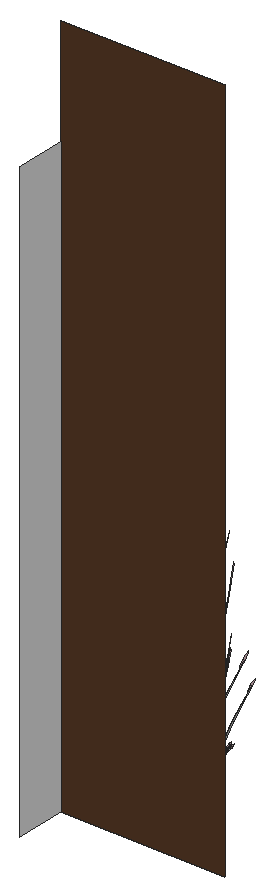
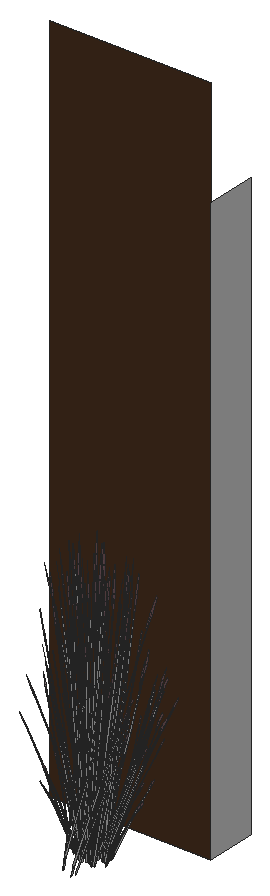
# SketchUp Ruby script. Lengths in inches.
U = 1.inch
M = Sketchup.active_model
def pt(a) = Geom::Point3d.new(a.map { |v| v * U })
def face(e, loops, mat)
  f = e.add_face(loops[0].map { |a| pt(a) })
  loops[1..].each { |l| e.add_face(l.map { |a| pt(a) }).erase! }
  f.material = f.back_material = mat if mat
  f
end
# faces: each face lists its corners as indices into pts; further lists are holes
def faces(e, pts, list, mat = nil) = list.each { |f| face(e, (f[0].is_a?(Array) ? f : [f]).map { |l| l.map { |i| pts[i] } }, mat) }
# xy, xz, yz: faces in a plane at the given z, y or x. An outline is a flat list of corners, or four numbers for a rectangle; further outlines are holes
def ring(l) = l.size == 4 ? [[l[0], l[1]], [l[2], l[1]], [l[2], l[3]], [l[0], l[3]]] : l.each_slice(2).to_a
def flat(e, list, mat, &to3) = list.each { |f| face(e, (f[0].is_a?(Array) ? f : [f]).map { |l| ring(l).map { |u, v| to3.(u, v) } }, mat) }
def xy(e, z, list, mat = nil) = flat(e, list, mat) { |x, y| [x, y, z] }
def xz(e, y, list, mat = nil) = flat(e, list, mat) { |x, z| [x, y, z] }
def yz(e, x, list, mat = nil) = flat(e, list, mat) { |y, z| [x, y, z] }
def lines(e, pts, list) = list.each { |a, b| e.add_line(pt(pts[a]), pt(pts[b])) }
# prism: a flat outline (further loops are holes) pulled along v
def prism(e, loops, v, mat = nil)
  f = face(e, loops, mat); d = Geom::Vector3d.new(v.map { |x| x * U })
  f.pushpull(f.normal.samedirection?(d) ? d.length : -d.length)
end
def box(e, o, s, mat = nil) = prism(e, [[o, [o[0] + s[0], o[1], o[2]], [o[0] + s[0], o[1] + s[1], o[2]], [o[0], o[1] + s[1], o[2]]]], [0, 0, s[2]], mat)
def at(x, y, z, deg = 0) = Geom::Transformation.translation(pt([x, y, z])) * Geom::Transformation.rotation(ORIGIN, Z_AXIS, deg.degrees)
def axes(o, x, y, z) = Geom::Transformation.new([*x, 0, *y, 0, *z, 0, *pt(o).to_a, 1])
def part(name) = M.definitions.add(name)
# library, detail: a bought-in or finely detailed component or shape, given as its bounding box
def library(name, o, s) = part(name).tap { |d| box(d.entities, o, s) }
def detail(e, o, s) = box(e.add_group.entities, o, s)
def put(e, d, t, mat = nil) = e.add_instance(d, t).tap { |i| i.material = mat if mat }
def group(e, t, mat = nil) = e.add_group.tap { |g| g.transformation = t; g.material = mat if mat }.entities
root = M.entities
M.materials.add("LightPink_Translucent").color = [144, 107, 117]
M.materials["LightPink_Translucent"].alpha = 0.75
M.materials.add("Wood_Veneer_15_1K").color = [81, 54, 35]
M.materials.add("[_0053_Ivory_]").color = [200, 200, 200]
c1 = part("blade")
p = [[2.15,0.21,22],[0,0.17,0],[0.09,0.45,0],[2.18,0.31,22],[2.29,0.31,22],[0.38,0.45,0],
  [2.48,0.24,33],[2.49,0.24,33],[2.48,0.22,33]]
faces(c1.entities,p,[[0,1,2,3],[4,5,2,3],[6,3,4,7],[8,0,3,6]])
c2 = part("seeds")
p = [[0.3,-0.1,1.38],[-0.01,-0.03,1.59],[-0.01,-0.03,0.03],[0.14,-0.07,-0.07],[0.29,-0.03,3],[0.15,0.01,3.11]]
faces(c2.entities,p,[[0,1,2,3],[1,0,4,5]],"LightPink_Translucent")
c3 = part("blade with seeds")
put(c3.entities,c1,at(0,0,0))
put(c3.entities,c2,axes([2.4,0.25,30.99],[1.5799,-0.05474,1.17369],[-0.12525,1.92788,0.29478],[-0.07173,-0.02425,1.56792]))
xz(root,269.15,[[617.51,252,653.51,408]],"Wood_Veneer_15_1K")
yz(root,617.51,[[257.92,252,269.15,384]],"[_0053_Ivory_]")
put(root,c3,axes([630.49,281.87,255.53],[0.13883,0.2019,1.71376],[-0.64153,0.16998,0.13857],[-0.14499,-0.31697,0.73262]),"[_0053_Ivory_]")
put(root,c3,axes([632.98,281.57,254.24],[-0.17264,0.12729,1.43002],[-0.51703,-0.22279,-0.30754],[0.09584,-0.27707,0.61141]),"[_0053_Ivory_]")
put(root,c3,axes([632.2,282.02,256.63],[-0.28988,-0.51132,-0.71045],[0.59671,-0.28496,0.08574],[-0.06778,-0.24706,1.00501]),"[_0053_Ivory_]")
put(root,c3,axes([630.3125,281.33,254.24],[-0.03678,0.20572,1.43002],[-0.53767,0.17221,-0.30754],[-0.12568,-0.26589,0.61141]),"[_0053_Ivory_]")
put(root,c3,axes([631.7,280.88,253.15],[-0.10187,0.02266,1.76342],[-0.56336,-0.25503,-0.26939],[0.00945,-0.21273,0.30037]),"[_0053_Ivory_]")
put(root,c3,axes([633.4,282.52,256.63],[0.0158,-0.58168,-0.71045],[0.66548,0.03907,0.08574],[0.07023,-0.24643,1.00501]),"[_0053_Ivory_]")
put(root,c3,axes([632.25,281.58,256.18],[0.1831,-0.48359,-0.35414],[0.53419,0.14105,0.4572],[-0.04898,-0.1947,0.87481]),"[_0053_Ivory_]")
put(root,c3,axes([632.65,282.22,255.53],[-0.11309,0.21615,1.71376],[-0.47441,-0.44731,0.13857],[0.21402,-0.27879,0.73262]),"[_0053_Ivory_]")
put(root,c3,axes([631.98,281.91,256.33],[-0.59704,-0.15764,-0.51099],[0.20464,-0.54049,-0.3958],[-0.05475,-0.21761,0.97773]),"[_0053_Ivory_]")
put(root,c3,axes([632.35,280.5625,254.42],[0.07791,0.3667,1.1486],[-0.43222,-0.2031,0.84392],[0.04651,-0.18776,0.25299]),"[_0053_Ivory_]")
put(root,c3,axes([633.27,282.32,256.33],[-0.43478,-0.42253,-0.51099],[0.45929,-0.37004,-0.3958],[0.06615,-0.21468,0.97773]),"[_0053_Ivory_]")
put(root,c3,axes([633.68,282.17,256.18],[0.41095,-0.33109,-0.35414],[0.38901,0.37805,0.4572],[0.05919,-0.19208,0.87481]),"[_0053_Ivory_]")
put(root,c3,axes([630.125,281,254.42],[0.31682,0.21887,1.1486],[-0.4614,0.13157,0.84392],[-0.09872,-0.16821,0.25299]),"[_0053_Ivory_]")
put(root,c3,axes([630.89,282.16,256.63],[-0.51789,-0.30395,-0.71045],[0.36805,-0.53263,0.08574],[-0.18764,-0.18149,1.00501]),"[_0053_Ivory_]")
put(root,c3,axes([630.71,281.76,256.18],[-0.0938,-0.50652,-0.35414],[0.53623,-0.13375,0.4572],[-0.14403,-0.14515,0.87481]),"[_0053_Ivory_]")
put(root,c3,axes([629.875,281.66,253.15],[-0.05883,0.08284,1.76342],[-0.59454,0.17861,-0.26939],[-0.14363,-0.16248,0.30037]),"[_0053_Ivory_]")
put(root,c3,axes([630.86,283.9375,253.75],[-0.24943,-0.64486,-0.69835],[0.71849,-0.23224,-0.18329],[-0.02757,-0.21836,1.54149]),"[_0053_Ivory_]")
put(root,c3,axes([629.56,282.5,255.53],[0.2256,0.10835,1.71376],[-0.46687,0.45453,0.13857],[-0.29098,-0.20505,0.73262]),"[_0053_Ivory_]")
put(root,c3,axes([634.19,281.97,253.15],[-0.0909,-0.04954,1.76342],[-0.2335,-0.55347,-0.26939],[0.15752,-0.1502,0.30037]),"[_0053_Ivory_]")
put(root,c3,axes([630.65,282.18,256.33],[-0.59932,0.14948,-0.51099],[-0.10484,-0.56611,-0.3958],[-0.16097,-0.16223,0.97773]),"[_0053_Ivory_]")
put(root,c3,axes([634.1875,283.53,256.63],[0.31725,-0.49618,-0.71045],[0.55593,0.35263,0.08574],[0.18942,-0.17977,1.00501]),"[_0053_Ivory_]")
put(root,c3,axes([630.76,282.08,254.03],[-0.37973,-0.63014,0],[0.6353,-0.35142,-0.51607],[0.14469,-0.08004,1.63711]),"[_0053_Ivory_]")
put(root,c3,axes([634.17,283.3,256.33],[-0.15602,-0.5742,-0.51099],[0.59087,-0.10045,-0.3958],[0.16933,-0.15423,0.97773]),"[_0053_Ivory_]")
put(root,c3,axes([631.59,281.32,253.78],[-0.4197,0.36076,-0.03893],[-0.38456,-0.39511,-0.17649],[-0.02707,-0.11196,0.58215]),"[_0053_Ivory_]")
put(root,c3,axes([632.13,285.6,254.98],[0.52485,0.25358,1.51261],[-0.51417,0.54629,0.59816],[-0.23031,-0.32378,1.26806]),"[_0053_Ivory_]")
put(root,c3,axes([629.39,283.85,253.67],[0,-0.62885,-0.49651],[0.67951,0,0],[0,-0.14322,1.57504]),"[_0053_Ivory_]")
put(root,c3,axes([631.27,281.99,253.67],[0.56842,-0.31443,-0.49651],[0.33976,0.56381,0],[0.12946,-0.07161,1.57504]),"[_0053_Ivory_]")
put(root,c3,axes([634.65,283.07,254.24],[-0.21697,-0.01863,1.43002],[-0.22228,-0.49966,-0.30754],[0.26655,-0.14135,0.61141]),"[_0053_Ivory_]")
put(root,c3,axes([631.95,283.28,253.71],[0.40909,-0.47266,-0.62353],[0.50819,0.4286,-0.16365],[0.16393,-0.11791,1.37633]),"[_0053_Ivory_]")
put(root,c3,axes([634.9,282.15,254.42],[-0.2023,0.32011,1.1486],[-0.17388,-0.43009,0.84392],[0.16708,-0.10777,0.25299]),"[_0053_Ivory_]")
put(root,c3,axes([634.61,283.36,256.18],[0.52868,-0.08987,-0.35414],[0.1396,0.51376,0.4572],[0.1515,-0.13799,0.87481]),"[_0053_Ivory_]")
put(root,c3,axes([631.24,284.1,253.86],[0.29468,-0.56664,-0.44739],[0.61229,0.27271,0.21531],[0,-0.13062,1.43643]),"[_0053_Ivory_]")
put(root,c3,axes([629.47,282.65,256.18],[-0.34557,-0.39372,-0.35414],[0.39459,-0.37271,0.4572],[-0.20048,-0.05671,0.87481]),"[_0053_Ivory_]")
put(root,c3,axes([631.5,283.82,254.32],[-0.07077,-0.71755,-0.29095],[0.73712,-0.04339,-0.50002],[0.1298,-0.09558,1.59708]),"[_0053_Ivory_]")
put(root,c3,axes([629.68,283.86,253.68],[0.42396,-0.39235,-0.30978],[0.42396,0.39235,0.30978],[0,-0.12637,1.38974]),"[_0053_Ivory_]")
put(root,c3,axes([629.51,281.98,253.78],[-0.1752,0.51349,-0.03893],[-0.53924,-0.15795,-0.17649],[-0.08187,-0.08399,0.58215]),"[_0053_Ivory_]")
put(root,c3,axes([631.16,284.58,254.32],[-0.68399,-0.30005,-0.29095],[0.32934,-0.63331,-0.50002],[-0.0215,-0.15549,1.59708]),"[_0053_Ivory_]")
put(root,c3,axes([629.22,284.32,254.03],[-0.75945,0,0],[0,-0.70283,-0.51607],[0,-0.16007,1.63711]),"[_0053_Ivory_]")
put(root,c3,axes([629.35,283.07,254.24],[0.11858,0.17508,1.43002],[-0.27325,0.4759,-0.30754],[-0.28057,-0.11375,0.61141]),"[_0053_Ivory_]")
put(root,c3,axes([631.41,282.23,253.68],[0.56663,0.1556,-0.30978],[-0.14267,0.54795,0.30978],[0.11423,-0.06319,1.38974]),"[_0053_Ivory_]")
put(root,c3,axes([629.83,282.91,256.63],[-0.60713,-0.01514,-0.71045],[0.04078,-0.63759,0.08574],[-0.25721,-0.06729,1.00501]),"[_0053_Ivory_]")
put(root,c3,axes([629.8,284.14,253.98],[-0.56493,0.5287,0.30756],[-0.56528,-0.52313,-0.36492],[-0.01973,-0.15014,1.64885]),"[_0053_Ivory_]")
put(root,c3,axes([631.6,284.39,254.09],[0.68433,0.30479,0.24065],[-0.32934,0.63331,0.50002],[0,-0.14599,1.60543]),"[_0053_Ivory_]")
put(root,c3,axes([631.33,285.24,254.09],[0.16098,-0.74515,-0.23429],[0.76326,0.12989,0.51271],[-0.13337,-0.1029,1.5644]),"[_0053_Ivory_]")
put(root,c3,axes([629.63,283.04,256.33],[-0.44101,0.41656,-0.51099],[-0.38623,-0.44004,-0.3958],[-0.22407,-0.06338,0.97773]),"[_0053_Ivory_]")
put(root,c3,axes([628.64,283.59,254.42],[0.38775,-0.045,1.1486],[-0.24596,0.39648,0.84392],[-0.19161,-0.05948,0.25299]),"[_0053_Ivory_]")
put(root,c3,axes([631.38,283.96,254.37],[-0.65953,0.03882,0.44739],[-0.05964,-0.64439,-0.21531],[0.11807,-0.06531,1.43643]),"[_0053_Ivory_]")
put(root,c3,axes([629.68,284.43,254.13],[0,0.62885,0.49651],[-0.67951,0,0],[0,-0.14322,1.57504]),"[_0053_Ivory_]")
put(root,c3,axes([634.45,284.57,256.33],[0.16454,-0.57202,-0.51099],[0.56413,0.19607,-0.3958],[0.22713,-0.05245,0.97773]),"[_0053_Ivory_]")
put(root,c3,axes([633.55,282.24,254.03],[0.37973,-0.63014,0],[0.6353,0.35142,-0.51607],[0.14469,0.08004,1.63711]),"[_0053_Ivory_]")
put(root,c3,axes([629.08,283.49,255.53],[0.25192,-0.01424,1.71376],[-0.16712,0.61729,0.13857],[-0.35901,-0.03818,0.73262]),"[_0053_Ivory_]")
put(root,c3,axes([631.28,284.9375,253.86],[-0.36485,-0.52782,-0.44739],[0.55265,-0.37168,0.21531],[-0.11807,-0.06531,1.43643]),"[_0053_Ivory_]")
put(root,c3,axes([631.36,284.19,254.01],[0.26406,0.70318,0.45755],[-0.7545,0.24452,0.17955],[0.00922,-0.12921,1.58856]),"[_0053_Ivory_]")
put(root,c3,axes([635.05,284.73,253.64],[-0.39118,0.07547,1.41583],[-0.06226,-0.6007,0.08104],[0.27398,-0.09092,0.80566]),"[_0053_Ivory_]")
put(root,c3,axes([635.76,284.2,253.91],[-0.37654,-0.40212,-0.06488],[0.4124,-0.36845,-0.29416],[0.11685,-0.02594,0.97024]),"[_0053_Ivory_]")
put(root,c3,axes([631.22,284.75,254.37],[-0.29468,0.56664,0.44739],[-0.61229,-0.27271,-0.21531],[0,-0.13062,1.43643]),"[_0053_Ivory_]")
put(root,c3,axes([632.31,284.25,253.86],[0,-0.72763,0],[0.75945,0,0],[0,0,1.79456]),"[_0053_Ivory_]")
put(root,c3,axes([633.23,282.57,254.13],[-0.56842,-0.31443,0.49651],[0.33976,-0.56381,0],[0.12946,0.07161,1.57504]),"[_0053_Ivory_]")
put(root,c3,axes([634.34,284.78,256.63],[0.53369,-0.27773,-0.71045],[0.29743,0.5717,0.08574],[0.25786,-0.06494,1.00501]),"[_0053_Ivory_]")
put(root,c3,axes([630.95,285.14,253.71],[-0.63179,-0.1031,-0.62353],[0.13332,-0.63596,-0.16365],[-0.18854,-0.07706,1.37633]),"[_0053_Ivory_]")
put(root,c3,axes([631.95,283.79,254.01],[-0.50358,0.57069,0.45755],[-0.59827,-0.50377,0.17955],[0.1214,-0.05695,1.58856]),"[_0053_Ivory_]")
put(root,c3,axes([632.5,284.82,253.95],[-0.56493,-0.54126,-0.06131],[0.56528,-0.54159,0],[-0.01973,-0.0189,1.75571]),"[_0053_Ivory_]")
put(root,c3,axes([631.07,282.85,254.13],[-0.17545,0.62497,0.17642],[-0.64204,-0.17686,0.35086],[0.11091,-0.00304,1.60407]),"[_0053_Ivory_]")
put(root,c3,axes([630.81,283.36,253.25],[-0.59782,0.25177,1.28929],[-0.19028,-0.72239,0.50096],[0.36709,0.01202,1.46642]),"[_0053_Ivory_]")
put(root,c3,axes([632.41,283.55,254.27],[0.11717,-0.56122,0.1448],[0.57245,0.09742,-0.41347],[0.10418,0.05763,1.26744]),"[_0053_Ivory_]")
put(root,c3,axes([631.42,284.88,254.01],[0.76764,0.13249,0.45755],[-0.15622,0.74829,0.17955],[-0.11218,-0.07226,1.58856]),"[_0053_Ivory_]")
put(root,c3,axes([635.48,284.34,253.15],[-0.03174,-0.09547,1.76342],[0.22015,-0.55846,-0.26939],[0.22208,-0.00803,0.30037]),"[_0053_Ivory_]")
put(root,c3,axes([628.92,284.24,253.15],[0.0154,0.09911,1.76342],[-0.31051,0.51756,-0.26939],[-0.22056,-0.02609,0.30037]),"[_0053_Ivory_]")
put(root,c3,axes([632.17,283.7,254.37],[-0.36485,-0.52782,0.44739],[0.55265,-0.37168,-0.21531],[0.11807,0.06531,1.43643]),"[_0053_Ivory_]")
put(root,c3,axes([630.28,286.11,253.68],[-0.14267,-0.54795,-0.30978],[0.56663,-0.1556,0.30978],[-0.11423,-0.06319,1.38974]),"[_0053_Ivory_]")
put(root,c3,axes([631.01,286.08,254.13],[0.65264,-0.16691,0.17642],[0.16115,0.62115,0.35086],[-0.05821,-0.0905,1.60407]),"[_0053_Ivory_]")
put(root,c3,axes([632.35,283.73,254.32],[0.61322,-0.4175,-0.29095],[0.40778,0.58992,-0.50002],[0.1513,0.05991,1.59708]),"[_0053_Ivory_]")
put(root,c3,axes([634.79,284.83,256.18],[0.50475,0.17543,-0.35414],[-0.14722,0.5118,0.4572],[0.20322,-0.04693,0.87481]),"[_0053_Ivory_]")
put(root,c3,axes([630.125,286.34,253.67],[-0.56842,-0.31443,-0.49651],[0.33976,-0.56381,0],[-0.12946,-0.07161,1.57504]),"[_0053_Ivory_]")
put(root,c3,axes([633.9,282.62,253.67],[0.56842,0.31443,-0.49651],[-0.33976,0.56381,0],[0.12946,0.07161,1.57504]),"[_0053_Ivory_]")
put(root,c3,axes([628.86,284.02,256.18],[-0.50475,-0.17543,-0.35414],[0.14722,-0.5118,0.4572],[-0.20322,0.04693,0.87481]),"[_0053_Ivory_]")
put(root,c3,axes([632.82,284.42,253.86],[0.67951,0,0],[0,0.65103,0],[0,0,1.78407]),"[_0053_Ivory_]")
put(root,c3,axes([631.67,285.24,254.32],[-0.61322,0.4175,-0.29095],[-0.40778,-0.58992,-0.50002],[-0.1513,-0.05991,1.59708]),"[_0053_Ivory_]")
put(root,c3,axes([633.01,282.89,254.13],[-0.65264,0.16691,0.17642],[-0.16115,-0.62115,0.35086],[0.05821,0.0905,1.60407]),"[_0053_Ivory_]")
put(root,c3,axes([633.42,284.2,255.53],[-0.25192,0.01424,1.71376],[0.16712,-0.61729,0.13857],[0.35901,0.03818,0.73262]),"[_0053_Ivory_]")
put(root,c3,axes([633.74,282.86,253.68],[0.14267,0.54795,-0.30978],[-0.56663,0.1556,0.30978],[0.11423,0.06319,1.38974]),"[_0053_Ivory_]")
put(root,c3,axes([632.6,284.08,254.03],[-0.76764,-0.13249,0.49198],[0.15622,-0.74829,0.19306],[0.11218,0.07226,1.70813]),"[_0053_Ivory_]")
put(root,c3,axes([631.99,285.93,253.86],[-0.19817,-0.54216,0],[0.56587,-0.18986,0],[0,0,1.54371]),"[_0053_Ivory_]")
put(root,c3,axes([631.61,285.42,254.27],[-0.11717,0.56122,0.1448],[-0.57245,-0.09742,-0.41347],[-0.10418,-0.05763,1.26744]),"[_0053_Ivory_]")
put(root,c3,axes([632.73,285.86,253.84],[0.63764,-0.21337,-0.19198],[0.22406,0.61462,0.00008],[0.07038,-0.02358,1.73897]),"[_0053_Ivory_]")
put(root,c3,axes([632.95,286.11,254.13],[0.17545,-0.62497,0.17642],[0.64204,0.17686,0.35086],[-0.11091,0.00304,1.60407]),"[_0053_Ivory_]")
put(root,c3,axes([632.81,284.69,253.87],[0.42396,0.40619,0],[-0.42396,0.40619,0],[0,0,1.69266]),"[_0053_Ivory_]")
put(root,c3,axes([630.4,283.93,255],[0.17264,-0.09097,1.77064],[0.05953,0.63516,0.13857],[-0.37394,0.08428,0.63284]),"[_0053_Ivory_]")
put(root,c3,axes([633.95,284.52,254.13],[-0.47719,-0.45806,0.17642],[0.48088,-0.44429,0.35086],[-0.0527,0.09355,1.60407]),"[_0053_Ivory_]")
put(root,c3,axes([633.07,283.83,253.71],[0.63179,0.1031,-0.62353],[-0.13332,0.63596,-0.16365],[0.18854,0.07706,1.37633]),"[_0053_Ivory_]")
put(root,c3,axes([635.86,284.9375,254.42],[-0.37526,0.10382,1.1486],[0.17664,-0.42906,0.84392],[0.19907,0.02936,0.25299]),"[_0053_Ivory_]")
put(root,c3,axes([631.85,286.18,253.85],[-0.61229,-0.28233,0],[0.29468,-0.58663,0],[0,0,1.62707]),"[_0053_Ivory_]")
put(root,c3,axes([632.36,285.43,254.12],[-0.59306,-0.50614,-0.25192],[0.49904,-0.56836,0.5513],[-0.1597,0.05921,1.68216]),"[_0053_Ivory_]")
put(root,c3,axes([630.8,286.4,254.13],[0.56842,0.31443,0.49651],[-0.33976,0.56381,0],[-0.12946,-0.07161,1.57504]),"[_0053_Ivory_]")
put(root,c3,axes([632.8,284.22,254.37],[0.29468,-0.56664,0.44739],[0.61229,0.27271,-0.21531],[0,0.13062,1.43643]),"[_0053_Ivory_]")
put(root,c3,axes([632.6875,284.54,253.95],[0,0.72727,-0.05637],[-0.75945,0,0],[0,0.02286,1.79368]),"[_0053_Ivory_]")
put(root,c3,axes([629.21,284.28,256.33],[-0.16454,0.57202,-0.51099],[-0.56413,-0.19607,-0.3958],[-0.22713,0.05245,0.97773]),"[_0053_Ivory_]")
put(root,c3,axes([632.74,284.03,253.86],[0.36485,0.52782,-0.44739],[-0.55265,0.37168,0.21531],[0.11807,0.06531,1.43643]),"[_0053_Ivory_]")
put(root,c3,axes([635.21,286.26,255.58],[-0.11624,-0.52862,-0.03492],[0.54943,-0.12153,-0.15832],[0.11473,0.03351,0.52218]),"[_0053_Ivory_]")
put(root,c3,axes([630.47,286.72,254.03],[-0.37973,0.63014,0],[-0.6353,-0.35142,-0.51607],[-0.14469,-0.08004,1.63711]),"[_0053_Ivory_]")
put(root,c3,axes([634.35,284.54,254.13],[0,-0.62885,0.49651],[0.67951,0,0],[0,0.14322,1.57504]),"[_0053_Ivory_]")
put(root,c3,axes([632.65,285.01,254.37],[0.65953,-0.03882,0.44739],[0.05964,0.64439,-0.21531],[-0.11807,0.06531,1.43643]),"[_0053_Ivory_]")
put(root,c3,axes([633.06,284.35,254.27],[0.56587,-0.18339,0.1448],[0.19817,0.52368,-0.41347],[0,0.11525,1.26744]),"[_0053_Ivory_]")
put(root,c3,axes([630.49,291.7,255.53],[0.13883,0.2019,1.71376],[-0.64153,0.16998,0.13857],[-0.14499,-0.31697,0.73262]),"[_0053_Ivory_]")
put(root,c3,axes([632.06,285.32,253.86],[-0.65953,0.03882,-0.44739],[-0.05964,-0.64439,0.21531],[-0.11807,0.06531,1.43643]),"[_0053_Ivory_]")
put(root,c3,axes([632.98,291.41,254.24],[-0.17264,0.12729,1.43002],[-0.51703,-0.22279,-0.30754],[0.09584,-0.27707,0.61141]),"[_0053_Ivory_]")
put(root,c3,axes([635.16,285.625,254.24],[-0.14627,-0.15466,1.43002],[0.19032,-0.51164,-0.30754],[0.29594,0.06931,0.61141]),"[_0053_Ivory_]")
put(root,c3,axes([632.2,291.85,256.63],[-0.28988,-0.51132,-0.71045],[0.59671,-0.28496,0.08574],[-0.06778,-0.24706,1.00501]),"[_0053_Ivory_]")
put(root,c3,axes([630.3125,291.17,254.24],[-0.03678,0.20572,1.43002],[-0.53767,0.17221,-0.30754],[-0.12568,-0.26589,0.61141]),"[_0053_Ivory_]")
put(root,c3,axes([632.55,286.1875,253.86],[0.61229,0.28233,0],[-0.29468,0.58663,0],[0,0,1.74954]),"[_0053_Ivory_]")
put(root,c3,axes([631.7,290.72,253.15],[-0.10187,0.02266,1.76342],[-0.56336,-0.25503,-0.26939],[0.00945,-0.21273,0.30037]),"[_0053_Ivory_]")
put(root,c3,axes([632.79,286.8125,253.85],[-0.37499,-0.63235,-0.05142],[0.6353,-0.35142,0.51607],[-0.15655,0.0602,1.6363]),"[_0053_Ivory_]")
put(root,c3,axes([632.66,285.28,254.27],[0.44871,0.37783,0.1448],[-0.37428,0.42627,-0.41347],[-0.10418,0.05763,1.26744]),"[_0053_Ivory_]")
